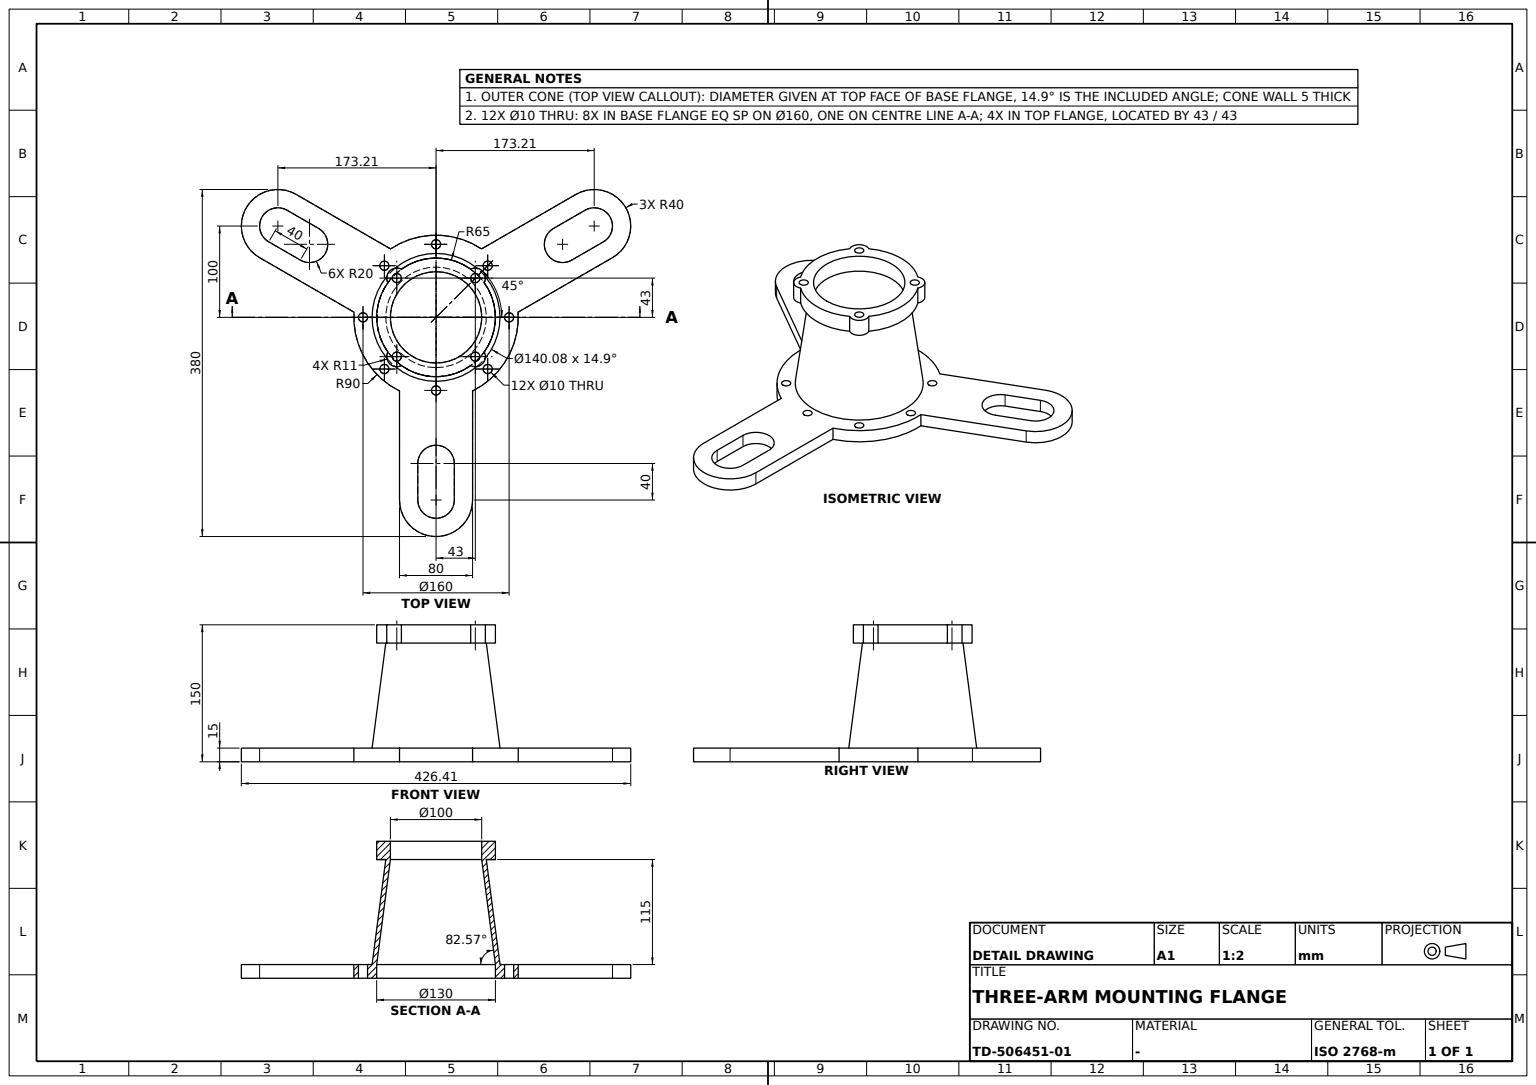
solid
v1 (85,0,0)
e1 v1 v1 CIRCLE(AX(P(80,0,0),D(0,0,1),D(1,0,0)),5)
v2 (85,0,15)
e2 v2 v2 CIRCLE(AX(P(80,0,15),D(0,0,1),D(1,0,0)),5)
face CYL(AX(P(80,0,7.5),D(0,0,1),D(1,0,0)),5) rev [-e1] [e2]
v3 (-134.641016,153.205081,0)
v4 (-134.641016,153.205081,15)
e3 v3 v4 LINE
v5 (-65.358984,193.205081,15)
e4 v5 v4 CIRCLE(AX(P(-100,173.205081,15),D(0,0,1),D(1,0,0)),40)
v6 (-65.358984,193.205081,0)
e5 v6 v5 LINE
e6 v6 v3 CIRCLE(AX(P(-100,173.205081,0),D(0,0,1),D(1,0,0)),40)
face CYL(AX(P(-100,173.205081,7.5),D(0,0,1),D(1,0,0)),40) [e3 -e4 -e5 e6]
v7 (160,-20,0)
v8 (200,-20,0)
e7 v7 v8 LINE
v9 (160,-20,15)
e8 v7 v9 LINE
v10 (200,-20,15)
e9 v9 v10 LINE
e10 v8 v10 LINE
face PLANE(AX(P(160,-20,0),D(0,-1,0),D(1,0,0))) rev [-e7 e8 e9 -e10]
v11 (-134.641016,-153.205081,0)
v12 (-65.358984,-193.205081,0)
e11 v11 v12 CIRCLE(AX(P(-100,-173.205081,0),D(0,0,1),D(1,0,0)),40)
v13 (-65.358984,-193.205081,15)
e12 v12 v13 LINE
v14 (-134.641016,-153.205081,15)
e13 v14 v13 CIRCLE(AX(P(-100,-173.205081,15),D(0,0,1),D(1,0,0)),40)
e14 v11 v14 LINE
face CYL(AX(P(-100,-173.205081,7.5),D(0,0,1),D(1,0,0)),40) [e11 e12 -e13 -e14]
v15 (160,20,0)
v16 (200,20,0)
e15 v15 v16 LINE
v17 (200,20,15)
e16 v16 v17 LINE
v18 (160,20,15)
e17 v18 v17 LINE
e18 v15 v18 LINE
face PLANE(AX(P(160,20,0),D(0,-1,0),D(1,0,0))) [e15 e16 -e17 -e18]
v19 (61.568542,-56.568542,15)
e19 v19 v19 CIRCLE(AX(P(56.568542,-56.568542,15),D(0,0,1),D(1,0,0)),5)
v20 (61.568542,-56.568542,0)
e20 v20 v20 CIRCLE(AX(P(56.568542,-56.568542,0),D(0,0,1),D(1,0,0)),5)
face CYL(AX(P(56.568542,-56.568542,7.5),D(0,0,1),D(1,0,0)),5) rev [e19] [-e20]
e21 v15 v7 CIRCLE(AX(P(160,0,0),D(0,0,1),D(1,0,0)),20)
e22 v18 v9 CIRCLE(AX(P(160,0,15),D(0,0,1),D(1,0,0)),20)
face CYL(AX(P(160,0,7.5),D(0,0,1),D(1,0,0)),20) rev [-e21 e18 e22 -e8]
v21 (-5.670273,89.8212,0)
e23 v21 v6 LINE
v22 (-5.670273,89.8212,15)
e24 v22 v5 LINE
e25 v21 v22 LINE
face PLANE(AX(P(-5.670273,89.8212,0),D(0.866025404,0.5,0),D(-0.5,0.866025404,0))) [e23 e5 -e24 -e25]
v23 (55.042354,0,130)
e26 v23 v23 CIRCLE(AX(P(0,0,130),D(0,0,1),D(1,0,0)),55.042354)
v24 (70.042354,0,15)
e27 v24 v24 CIRCLE(AX(P(0,0,15),D(0,0,1),D(1,0,0)),70.042354)
face CONE(AX(P(0,0,130),D(0,0,-1),D(1,0,0)),55.042353698,0.129702537) [-e26] [e27]
v25 (61.568542,56.568542,0)
e28 v25 v25 CIRCLE(AX(P(56.568542,56.568542,0),D(0,0,1),D(1,0,0)),5)
v26 (61.568542,56.568542,15)
e29 v26 v26 CIRCLE(AX(P(56.568542,56.568542,15),D(0,0,1),D(1,0,0)),5)
face CYL(AX(P(56.568542,56.568542,7.5),D(0,0,1),D(1,0,0)),5) rev [-e28] [e29]
v27 (-65,0,15)
e30 v27 v27 CIRCLE(AX(P(0,0,15),D(0,0,-1),D(-1,0,0)),65) rev
v28 (-50,0,130)
e31 v28 v28 CIRCLE(AX(P(0,0,130),D(0,0,-1),D(-1,0,0)),50) rev
face CONE(AX(P(0,0,130),D(0,0,-1),D(1,0,0)),50,0.129702537) rev [-e30] [e31]
v29 (-74.952305,49.8212,15)
e32 v29 v4 LINE
v30 (-74.952305,49.8212,0)
e33 v30 v3 LINE
e34 v30 v29 LINE
face PLANE(AX(P(-74.952305,49.8212,0),D(0.866025404,0.5,0),D(-0.5,0.866025404,0))) rev [e32 -e3 -e33 e34]
v31 (80.622577,40,15)
e35 v31 v22 CIRCLE(AX(P(0,0,15),D(0,0,1),D(1,0,0)),90)
v32 (80.622577,40,0)
e36 v32 v31 LINE
e37 v32 v21 CIRCLE(AX(P(0,0,0),D(0,0,1),D(1,0,0)),90)
face CYL(AX(P(0,0,7.5),D(0,0,1),D(1,0,0)),90) [e25 -e35 -e36 e37]
v33 (-82.679492,-183.205081,0)
v34 (-82.679492,-183.205081,15)
e38 v33 v34 LINE
v35 (-117.320508,-163.205081,0)
e39 v35 v33 CIRCLE(AX(P(-100,-173.205081,0),D(0,0,1),D(1,0,0)),20)
v36 (-117.320508,-163.205081,15)
e40 v35 v36 LINE
e41 v36 v34 CIRCLE(AX(P(-100,-173.205081,15),D(0,0,1),D(1,0,0)),20)
face CYL(AX(P(-100,-173.205081,7.5),D(0,0,1),D(1,0,0)),20) rev [-e38 -e39 e40 e41]
v37 (-62.679492,148.564065,0)
v38 (-62.679492,148.564065,15)
e42 v37 v38 LINE
v39 (-82.679492,183.205081,15)
e43 v38 v39 LINE
v40 (-82.679492,183.205081,0)
e44 v40 v39 LINE
e45 v37 v40 LINE
face PLANE(AX(P(-62.679492,148.564065,0),D(0.866025404,0.5,0),D(-0.5,0.866025404,0))) rev [e42 e43 -e44 -e45]
v41 (37.949109,-52.771822,130)
v42 (37.949109,-52.771822,150)
e46 v41 v42 LINE
v43 (-37.949109,-52.771822,150)
e47 v43 v42 CIRCLE(AX(P(0,0,150),D(0,0,1),D(1,0,0)),65)
v44 (-37.949109,-52.771822,130)
e48 v44 v43 LINE
e49 v44 v41 CIRCLE(AX(P(0,0,130),D(0,0,1),D(1,0,0)),65)
face CYL(AX(P(0,0,140),D(0,0,1),D(1,0,0)),65) [e46 -e47 -e48 e49]
v45 (48,43,130)
e50 v45 v45 CIRCLE(AX(P(43,43,130),D(0,0,1),D(1,0,0)),5)
v46 (48,43,150)
e51 v46 v46 CIRCLE(AX(P(43,43,150),D(0,0,1),D(1,0,0)),5)
face CYL(AX(P(43,43,140),D(0,0,1),D(1,0,0)),5) rev [-e50] [e51]
v47 (50,0,150)
e52 v47 v47 CIRCLE(AX(P(0,0,150),D(0,0,1),D(1,0,0)),50)
v48 (-38,43,150)
e53 v48 v48 CIRCLE(AX(P(-43,43,150),D(0,0,1),D(1,0,0)),5)
v49 (37.949109,52.771822,150)
v50 (-37.949109,52.771822,150)
e54 v49 v50 CIRCLE(AX(P(0,0,150),D(0,0,1),D(1,0,0)),65)
v51 (-52.771822,37.949109,150)
e55 v50 v51 CIRCLE(AX(P(-43,43,150),D(0,0,1),D(1,0,0)),11)
v52 (-52.771822,-37.949109,150)
e56 v51 v52 CIRCLE(AX(P(0,0,150),D(0,0,1),D(1,0,0)),65)
e57 v52 v43 CIRCLE(AX(P(-43,-43,150),D(0,0,1),D(1,0,0)),11)
v53 (52.771822,-37.949109,150)
e58 v42 v53 CIRCLE(AX(P(43,-43,150),D(0,0,1),D(1,0,0)),11)
v54 (52.771822,37.949109,150)
e59 v53 v54 CIRCLE(AX(P(0,0,150),D(0,0,1),D(1,0,0)),65)
e60 v54 v49 CIRCLE(AX(P(43,43,150),D(0,0,1),D(1,0,0)),11)
v55 (-38,-43,150)
e61 v55 v55 CIRCLE(AX(P(-43,-43,150),D(0,0,1),D(1,0,0)),5)
v56 (48,-43,150)
e62 v56 v56 CIRCLE(AX(P(43,-43,150),D(0,0,1),D(1,0,0)),5)
face PLANE(AX(P(0,0,150),D(0,0,1),D(1,0,0))) [-e52] [-e53] [e54 e55 e56 e57 e47 e58 e59 e60] [-e61] [-e51] [-e62]
v57 (-97.320508,128.564065,0)
v58 (-97.320508,128.564065,15)
e63 v57 v58 LINE
v59 (-117.320508,163.205081,0)
e64 v57 v59 LINE
v60 (-117.320508,163.205081,15)
e65 v59 v60 LINE
e66 v58 v60 LINE
face PLANE(AX(P(-97.320508,128.564065,0),D(0.866025404,0.5,0),D(-0.5,0.866025404,0))) [-e63 e64 e65 -e66]
v61 (48,-43,130)
e67 v61 v61 CIRCLE(AX(P(43,-43,130),D(0,0,1),D(1,0,0)),5)
face CYL(AX(P(43,-43,140),D(0,0,1),D(1,0,0)),5) rev [e62] [-e67]
v62 (-74.952305,-49.8212,15)
e68 v62 v14 LINE
v63 (-74.952305,-49.8212,0)
e69 v63 v62 LINE
e70 v63 v11 LINE
face PLANE(AX(P(-74.952305,-49.8212,0),D(-0.866025404,0.5,0),D(-0.5,-0.866025404,0))) [e14 -e68 -e69 e70]
v64 (-62.679492,-148.564065,15)
v65 (-97.320508,-128.564065,15)
e71 v64 v65 CIRCLE(AX(P(-80,-138.564065,15),D(0,0,1),D(1,0,0)),20)
v66 (-97.320508,-128.564065,0)
e72 v66 v65 LINE
v67 (-62.679492,-148.564065,0)
e73 v67 v66 CIRCLE(AX(P(-80,-138.564065,0),D(0,0,1),D(1,0,0)),20)
e74 v67 v64 LINE
face CYL(AX(P(-80,-138.564065,7.5),D(0,0,1),D(1,0,0)),20) rev [e71 -e72 -e73 e74]
v68 (65,0,0)
e75 v68 v68 CIRCLE(AX(P(0,0,0),D(0,0,1),D(1,0,0)),65)
face CYL(AX(P(0,0,140),D(0,0,1),D(1,0,0)),65) rev [-e75] [e30]
e76 v58 v38 CIRCLE(AX(P(-80,138.564065,15),D(0,0,1),D(1,0,0)),20)
e77 v57 v37 CIRCLE(AX(P(-80,138.564065,0),D(0,0,1),D(1,0,0)),20)
face CYL(AX(P(-80,138.564065,7.5),D(0,0,1),D(1,0,0)),20) rev [e63 e76 -e42 -e77]
v69 (-38,43,130)
e78 v69 v69 CIRCLE(AX(P(-43,43,130),D(0,0,1),D(1,0,0)),5)
face CYL(AX(P(-43,43,140),D(0,0,1),D(1,0,0)),5) rev [-e78] [e53]
v70 (-38,-43,130)
e79 v70 v70 CIRCLE(AX(P(-43,-43,130),D(0,0,1),D(1,0,0)),5)
face CYL(AX(P(-43,-43,140),D(0,0,1),D(1,0,0)),5) rev [e61] [-e79]
face CYL(AX(P(0,0,140),D(0,0,1),D(1,0,0)),50) rev [-e31] [e52]
v71 (52.771822,-37.949109,130)
e80 v41 v71 CIRCLE(AX(P(43,-43,130),D(0,0,1),D(1,0,0)),11)
e81 v71 v53 LINE
face CYL(AX(P(43,-43,140),D(0,0,1),D(1,0,0)),11) [-e58 -e46 e80 e81]
v72 (-5.670273,-89.8212,15)
v73 (80.622577,-40,15)
e82 v72 v73 CIRCLE(AX(P(0,0,15),D(0,0,1),D(1,0,0)),90)
v74 (-5.670273,-89.8212,0)
e83 v74 v72 LINE
v75 (80.622577,-40,0)
e84 v74 v75 CIRCLE(AX(P(0,0,0),D(0,0,1),D(1,0,0)),90)
e85 v75 v73 LINE
face CYL(AX(P(0,0,7.5),D(0,0,1),D(1,0,0)),90) [-e82 -e83 e84 e85]
v76 (-51.568542,-56.568542,15)
e86 v76 v76 CIRCLE(AX(P(-56.568542,-56.568542,15),D(0,0,1),D(1,0,0)),5)
v77 (-51.568542,-56.568542,0)
e87 v77 v77 CIRCLE(AX(P(-56.568542,-56.568542,0),D(0,0,1),D(1,0,0)),5)
face CYL(AX(P(-56.568542,-56.568542,7.5),D(0,0,1),D(1,0,0)),5) rev [e86] [-e87]
v78 (-51.568542,56.568542,0)
e88 v78 v78 CIRCLE(AX(P(-56.568542,56.568542,0),D(0,0,1),D(1,0,0)),5)
v79 (5,-80,0)
e89 v79 v79 CIRCLE(AX(P(0,-80,0),D(0,0,1),D(1,0,0)),5)
v80 (-75,0,0)
e90 v80 v80 CIRCLE(AX(P(-80,0,0),D(0,0,1),D(1,0,0)),5)
v81 (5,80,0)
e91 v81 v81 CIRCLE(AX(P(0,80,0),D(0,0,1),D(1,0,0)),5)
e92 v66 v35 LINE
e93 v67 v33 LINE
v82 (200,-40,0)
e94 v75 v82 LINE
e95 v74 v12 LINE
e96 v30 v63 CIRCLE(AX(P(0,0,0),D(0,0,1),D(1,0,0)),90)
v83 (200,40,0)
e97 v32 v83 LINE
e98 v82 v83 CIRCLE(AX(P(200,0,0),D(0,0,1),D(1,0,0)),40)
e99 v40 v59 CIRCLE(AX(P(-100,173.205081,0),D(0,0,1),D(1,0,0)),20)
e100 v8 v16 CIRCLE(AX(P(200,0,0),D(0,0,1),D(1,0,0)),20)
face PLANE(AX(P(0,0,0),D(0,0,1),D(1,0,0))) rev [e88] [e87] [e89] [e28] [e90] [e20] [e91] [e1] [e73 e92 e39 -e93] [-e94 -e84 e95 -e11 -e70 -e96 e33 -e6 -e23 -e37 e97 -e98] [e75] [e77 e45 e99 -e64] [e7 e100 -e15 e21]
v84 (-37.949109,52.771822,130)
v85 (-52.771822,37.949109,130)
e101 v84 v85 CIRCLE(AX(P(-43,43,130),D(0,0,1),D(1,0,0)),11)
e102 v85 v51 LINE
e103 v84 v50 LINE
face CYL(AX(P(-43,43,140),D(0,0,1),D(1,0,0)),11) [e101 e102 -e55 -e103]
v86 (5,-80,15)
e104 v86 v86 CIRCLE(AX(P(0,-80,15),D(0,0,1),D(1,0,0)),5)
face CYL(AX(P(0,-80,7.5),D(0,0,1),D(1,0,0)),5) rev [-e89] [e104]
v87 (52.771822,37.949109,130)
e105 v87 v54 LINE
e106 v71 v87 CIRCLE(AX(P(0,0,130),D(0,0,1),D(1,0,0)),65)
face CYL(AX(P(0,0,140),D(0,0,1),D(1,0,0)),65) [e105 -e59 -e81 e106]
v88 (37.949109,52.771822,130)
e107 v88 v49 LINE
e108 v88 v84 CIRCLE(AX(P(0,0,130),D(0,0,1),D(1,0,0)),65)
face CYL(AX(P(0,0,140),D(0,0,1),D(1,0,0)),65) [-e107 e108 e103 -e54]
v89 (200,40,15)
e109 v31 v89 LINE
e110 v83 v89 LINE
face PLANE(AX(P(80.622577,40,0),D(0,-1,0),D(1,0,0))) rev [e36 e109 -e110 -e97]
v90 (-51.568542,56.568542,15)
e111 v90 v90 CIRCLE(AX(P(-56.568542,56.568542,15),D(0,0,1),D(1,0,0)),5)
e112 v39 v60 CIRCLE(AX(P(-100,173.205081,15),D(0,0,1),D(1,0,0)),20)
v91 (200,-40,15)
e113 v73 v91 LINE
e114 v91 v89 CIRCLE(AX(P(200,0,15),D(0,0,1),D(1,0,0)),40)
e115 v29 v62 CIRCLE(AX(P(0,0,15),D(0,0,1),D(1,0,0)),90)
e116 v72 v13 LINE
e117 v65 v36 LINE
e118 v64 v34 LINE
v92 (-75,0,15)
e119 v92 v92 CIRCLE(AX(P(-80,0,15),D(0,0,1),D(1,0,0)),5)
e120 v10 v17 CIRCLE(AX(P(200,0,15),D(0,0,1),D(1,0,0)),20)
v93 (5,80,15)
e121 v93 v93 CIRCLE(AX(P(0,80,15),D(0,0,1),D(1,0,0)),5)
face PLANE(AX(P(0,0,15),D(0,0,1),D(1,0,0))) [-e2] [-e111] [-e104] [e66 -e112 -e43 -e76] [e113 e114 -e109 e35 e24 e4 -e32 e115 e68 e13 -e116 e82] [-e27] [-e86] [-e117 -e71 e118 -e41] [-e19] [-e119] [-e9 -e22 e17 -e120] [-e29] [-e121]
face CYL(AX(P(-80,0,7.5),D(0,0,1),D(1,0,0)),5) rev [e119] [-e90]
face CYL(AX(P(-56.568542,56.568542,7.5),D(0,0,1),D(1,0,0)),5) rev [-e88] [e111]
face CYL(AX(P(0,0,7.5),D(0,0,1),D(1,0,0)),90) [e96 e69 -e115 -e34]
v94 (-52.771822,-37.949109,130)
e122 v94 v44 CIRCLE(AX(P(-43,-43,130),D(0,0,1),D(1,0,0)),11)
e123 v94 v52 LINE
face CYL(AX(P(-43,-43,140),D(0,0,1),D(1,0,0)),11) [e122 e48 -e57 -e123]
face PLANE(AX(P(-97.320508,-128.564065,0),D(-0.866025404,0.5,0),D(-0.5,-0.866025404,0))) rev [-e40 -e92 e72 e117]
e124 v87 v88 CIRCLE(AX(P(43,43,130),D(0,0,1),D(1,0,0)),11)
face CYL(AX(P(43,43,140),D(0,0,1),D(1,0,0)),11) [-e105 e124 e107 -e60]
face PLANE(AX(P(-5.670273,-89.8212,0),D(-0.866025404,0.5,0),D(-0.5,-0.866025404,0))) rev [e83 e116 -e12 -e95]
face CYL(AX(P(200,0,7.5),D(0,0,1),D(1,0,0)),20) rev [-e16 -e100 e10 e120]
e125 v82 v91 LINE
face CYL(AX(P(200,0,7.5),D(0,0,1),D(1,0,0)),40) [-e114 -e125 e98 e110]
e126 v85 v94 CIRCLE(AX(P(0,0,130),D(0,0,1),D(1,0,0)),65)
face PLANE(AX(P(0,-50,130),D(0,0,1),D(1,0,0))) rev [-e49 -e122 -e126 -e101 -e108 -e124 -e106 -e80] [e26] [e79] [e78] [e67] [e50]
face CYL(AX(P(-100,173.205081,7.5),D(0,0,1),D(1,0,0)),20) rev [e44 e112 -e65 -e99]
face PLANE(AX(P(-62.679492,-148.564065,0),D(-0.866025404,0.5,0),D(-0.5,-0.866025404,0))) [-e118 -e74 e93 e38]
face PLANE(AX(P(80.622577,-40,0),D(0,-1,0),D(1,0,0))) [-e85 e94 e125 -e113]
face CYL(AX(P(0,80,7.5),D(0,0,1),D(1,0,0)),5) rev [-e91] [e121]
face CYL(AX(P(0,0,140),D(0,0,1),D(1,0,0)),65) [e126 e123 -e56 -e102]
